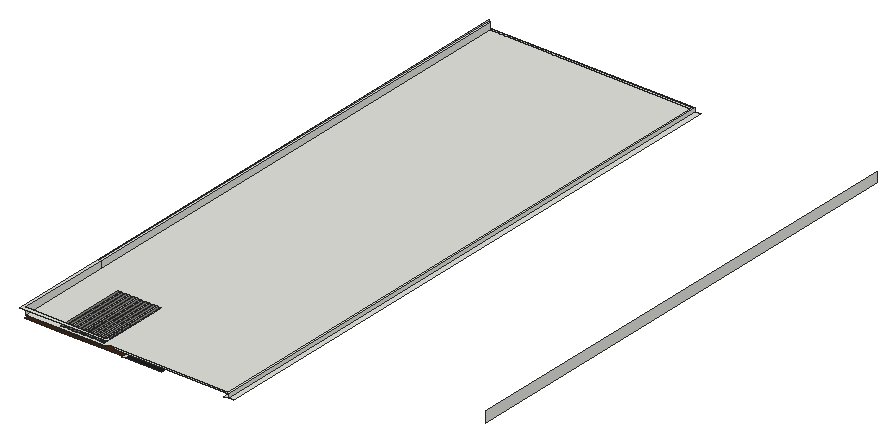
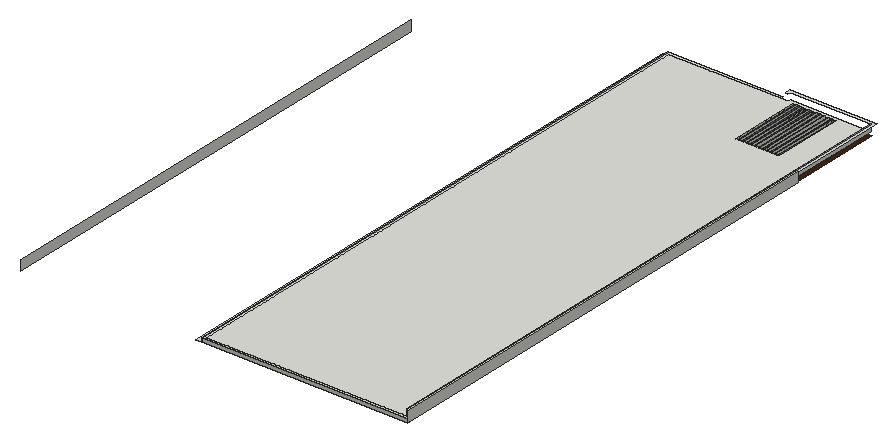
# SketchUp Ruby script. Lengths in inches.
U = 1.inch
M = Sketchup.active_model
def pt(a) = Geom::Point3d.new(a.map { |v| v * U })
def face(e, loops, mat)
  f = e.add_face(loops[0].map { |a| pt(a) })
  loops[1..].each { |l| e.add_face(l.map { |a| pt(a) }).erase! }
  f.material = f.back_material = mat if mat
  f
end
# faces: each face lists its corners as indices into pts; further lists are holes
def faces(e, pts, list, mat = nil) = list.each { |f| face(e, (f[0].is_a?(Array) ? f : [f]).map { |l| l.map { |i| pts[i] } }, mat) }
# xy, xz, yz: faces in a plane at the given z, y or x. An outline is a flat list of corners, or four numbers for a rectangle; further outlines are holes
def ring(l) = l.size == 4 ? [[l[0], l[1]], [l[2], l[1]], [l[2], l[3]], [l[0], l[3]]] : l.each_slice(2).to_a
def flat(e, list, mat, &to3) = list.each { |f| face(e, (f[0].is_a?(Array) ? f : [f]).map { |l| ring(l).map { |u, v| to3.(u, v) } }, mat) }
def xy(e, z, list, mat = nil) = flat(e, list, mat) { |x, y| [x, y, z] }
def xz(e, y, list, mat = nil) = flat(e, list, mat) { |x, z| [x, y, z] }
def yz(e, x, list, mat = nil) = flat(e, list, mat) { |y, z| [x, y, z] }
def lines(e, pts, list) = list.each { |a, b| e.add_line(pt(pts[a]), pt(pts[b])) }
# prism: a flat outline (further loops are holes) pulled along v
def prism(e, loops, v, mat = nil)
  f = face(e, loops, mat); d = Geom::Vector3d.new(v.map { |x| x * U })
  f.pushpull(f.normal.samedirection?(d) ? d.length : -d.length)
end
def box(e, o, s, mat = nil) = prism(e, [[o, [o[0] + s[0], o[1], o[2]], [o[0] + s[0], o[1] + s[1], o[2]], [o[0], o[1] + s[1], o[2]]]], [0, 0, s[2]], mat)
def at(x, y, z, deg = 0) = Geom::Transformation.translation(pt([x, y, z])) * Geom::Transformation.rotation(ORIGIN, Z_AXIS, deg.degrees)
def axes(o, x, y, z) = Geom::Transformation.new([*x, 0, *y, 0, *z, 0, *pt(o).to_a, 1])
def part(name) = M.definitions.add(name)
# library, detail: a bought-in or finely detailed component or shape, given as its bounding box
def library(name, o, s) = part(name).tap { |d| box(d.entities, o, s) }
def detail(e, o, s) = box(e.add_group.entities, o, s)
def put(e, d, t, mat = nil) = e.add_instance(d, t).tap { |i| i.material = mat if mat }
def group(e, t, mat = nil) = e.add_group.tap { |g| g.transformation = t; g.material = mat if mat }.entities
root = M.entities
M.materials.add("[Color M08]").color = [30, 30, 30]
M.materials.add("[Field Square Tile]").color = [211, 167, 108]
M.materials.add("[Granite Light Gray]").color = [149, 148, 144]
M.materials.add("[Wood Veneer 01]").color = [66, 38, 20]
xy(root,380.5,[[676.54,511.08,676.54,1825.82,228.78,1825.82,228.78,762.17,444.78,762.17,444.78,727.2,218.97,727.2,218.97,1835.625,686.35,1835.625,686.35,511.08],[444.78,511.08,453.7,589.83],[686.35,511.08,698.16,1835.625],[444.78,589.83,444.78,762.17,228.78,762.17,228.78,1825.82,676.54,1825.82,676.54,589.83,629.77,589.83,629.77,697.21,534.46,697.21,534.46,738.02,453.7,738.02,453.7,697.21,445.08,697.21,445.08,589.83],[445.08,589.83,453.7,697.21],
  [534.46,589.83,629.77,697.21],[453.7,697.21,534.46,738.02]])
xy(root,380.5,[[453.7,511.08,534.46,697.21]],"[Color M08]")
xy(root,380.5,[[[223.8,512.27,295.73,727.2],[240.83,666.01,242.35,666.38,243.73,667.14,244.86,668.22,245.67,669.56,246.1,671.0625,246.14,672.63,245.76,674.15,245.01,675.52,243.92,676.65,242.58,677.46,241.08,677.9,239.51,677.93,237.99,677.56,236.62,676.81,235.49,675.72,234.68,674.38,234.24,672.875,234.21,671.3125,234.58,669.79,235.34,668.42,236.42,667.29,237.76,666.48,239.27,666.04],[240.83,606.01,242.35,606.38,243.73,607.14,244.86,608.22,245.67,609.56,246.1,611.0625,246.14,612.63,245.76,614.15,245.01,615.52,243.92,616.65,242.58,617.46,241.08,617.9,239.51,617.93,237.99,617.56,236.62,616.81,235.49,615.72,234.68,614.38,234.24,612.875,234.21,611.3125,234.58,609.79,235.34,608.42,236.42,607.29,237.76,606.48,239.27,606.04],[240.83,554.26,242.35,554.63,243.73,555.39,244.86,556.47,245.67,557.81,246.1,559.3125,246.14,560.88,245.76,562.4,245.01,563.77,243.92,564.9,242.58,565.71,241.08,566.15,239.51,566.18,237.99,565.81,236.62,565.06,235.49,563.97,234.68,562.63,234.24,561.125,234.21,559.5625,234.58,558.04,235.34,556.67,236.42,555.54,237.76,554.73,239.27,554.29],[240.83,523.51,242.35,523.88,243.73,524.64,244.86,525.72,245.67,527.06,246.1,528.5625,246.14,530.13,245.76,531.65,245.01,533.02,243.92,534.15,242.58,534.96,241.08,535.4,239.51,535.43,237.99,535.06,236.62,534.31,235.49,533.22,234.68,531.88,234.24,530.375,234.21,528.8125,234.58,527.29,235.34,525.92,236.42,524.79,237.76,523.98,239.27,523.54],[280.58,666.01,282.1,666.38,283.48,667.14,284.61,668.22,285.42,669.56,285.85,671.0625,285.89,672.63,285.51,674.15,284.76,675.52,283.67,676.65,282.33,677.46,280.83,677.9,279.26,677.93,277.74,677.56,276.37,676.81,275.24,675.72,274.43,674.38,273.99,672.875,273.96,671.3125,274.33,669.79,275.09,668.42,276.17,667.29,277.51,666.48,279.02,666.04],[280.58,606.01,282.1,606.38,283.48,607.14,284.61,608.22,285.42,609.56,285.85,611.0625,285.89,612.63,285.51,614.15,284.76,615.52,283.67,616.65,282.33,617.46,280.83,617.9,279.26,617.93,277.74,617.56,276.37,616.81,275.24,615.72,274.43,614.38,273.99,612.875,273.96,611.3125,274.33,609.79,275.09,608.42,276.17,607.29,277.51,606.48,279.02,606.04],[280.58,554.26,282.1,554.63,283.48,555.39,284.61,556.47,285.42,557.81,285.85,559.3125,285.89,560.88,285.51,562.4,284.76,563.77,283.67,564.9,282.33,565.71,280.83,566.15,279.26,566.18,277.74,565.81,276.37,565.06,275.24,563.97,274.43,562.63,273.99,561.125,273.96,559.5625,274.33,558.04,275.09,556.67,276.17,555.54,277.51,554.73,279.02,554.29],[280.58,523.51,282.1,523.88,283.48,524.64,284.61,525.72,285.42,527.06,285.85,528.5625,285.89,530.13,285.51,531.65,284.76,533.02,283.67,534.15,282.33,534.96,280.83,535.4,279.26,535.43,277.74,535.06,276.37,534.31,275.24,533.22,274.43,531.88,273.99,530.375,273.96,528.8125,274.33,527.29,275.09,525.92,276.17,524.79,277.51,523.98,279.02,523.54]],[[295.73,512.27,444.78,727.2],[391.18,519.43,397.43,680.49],[382.06,519.43,388.31,680.49],[372.93,519.43,379.18,680.49],[363.81,519.43,370.06,680.49],[354.68,519.43,360.93,680.49],[345.56,519.43,351.81,680.49],[336.43,519.43,342.68,680.49],[327.31,519.43,333.56,680.49],[318.18,519.43,324.43,680.49],[309.06,519.43,315.31,680.49],[299.93,519.43,306.18,680.49]]],"[Wood Veneer 01]")
xy(root,381.875,[[240.83,554.26,239.27,554.29,237.76,554.73,236.42,555.54,235.34,556.67,234.58,558.04,234.21,559.5625,234.24,561.125,234.68,562.63,235.49,563.97,236.62,565.06,237.99,565.81,239.51,566.18,241.08,566.15,242.58,565.71,243.92,564.9,245.01,563.77,245.76,562.4,246.14,560.88,246.1,559.3125,245.67,557.81,244.86,556.47,243.73,555.39,242.35,554.63],[280.58,554.26,279.02,554.29,277.51,554.73,276.17,555.54,275.09,556.67,274.33,558.04,273.96,559.5625,273.99,561.125,274.43,562.63,275.24,563.97,276.37,565.06,277.74,565.81,279.26,566.18,280.83,566.15,282.33,565.71,283.67,564.9,284.76,563.77,285.51,562.4,285.89,560.88,285.85,559.3125,285.42,557.81,284.61,556.47,283.48,555.39,282.1,554.63],[240.83,606.01,239.27,606.04,237.76,606.48,236.42,607.29,235.34,608.42,234.58,609.79,234.21,611.3125,234.24,612.875,234.68,614.38,235.49,615.72,236.62,616.81,237.99,617.56,239.51,617.93,241.08,617.9,242.58,617.46,243.92,616.65,245.01,615.52,245.76,614.15,246.14,612.63,246.1,611.0625,245.67,609.56,244.86,608.22,243.73,607.14,242.35,606.38],[280.58,606.01,279.02,606.04,277.51,606.48,276.17,607.29,275.09,608.42,274.33,609.79,273.96,611.3125,273.99,612.875,274.43,614.38,275.24,615.72,276.37,616.81,277.74,617.56,279.26,617.93,280.83,617.9,282.33,617.46,283.67,616.65,284.76,615.52,285.51,614.15,285.89,612.63,285.85,611.0625,285.42,609.56,284.61,608.22,283.48,607.14,282.1,606.38],[240.83,666.01,239.27,666.04,237.76,666.48,236.42,667.29,235.34,668.42,234.58,669.79,234.21,671.3125,234.24,672.875,234.68,674.38,235.49,675.72,236.62,676.81,237.99,677.56,239.51,677.93,241.08,677.9,242.58,677.46,243.92,676.65,245.01,675.52,245.76,674.15,246.14,672.63,246.1,671.0625,245.67,669.56,244.86,668.22,243.73,667.14,242.35,666.38],
  [280.58,666.01,279.02,666.04,277.51,666.48,276.17,667.29,275.09,668.42,274.33,669.79,273.96,671.3125,273.99,672.875,274.43,674.38,275.24,675.72,276.37,676.81,277.74,677.56,279.26,677.93,280.83,677.9,282.33,677.46,283.67,676.65,284.76,675.52,285.51,674.15,285.89,672.63,285.85,671.0625,285.42,669.56,284.61,668.22,283.48,667.14,282.1,666.38]],"[Field Square Tile]")
xy(root,388.625,[[[225.31,510.87,408.63,510.87,408.63,517.43,680,517.43,680,1829.28,225.31,1829.28],[299.93,519.43,306.18,680.49],[309.06,519.43,315.31,680.49],[318.18,519.43,324.43,680.49],[327.31,519.43,333.56,680.49],[336.43,519.43,342.68,680.49],[345.56,519.43,351.81,680.49],[354.68,519.43,360.93,680.49],[363.81,519.43,370.06,680.49],[372.93,519.43,379.18,680.49],[382.06,519.43,388.31,680.49],[391.18,519.43,397.43,680.49]],[425.6875,511.08,686.35,511.08,686.35,1835.625,218.97,1835.625,225.31,1829.28,680,1829.28,680,517.43,425.6875,517.43]])
xy(root,403.8125,[[218.97,504.52,414.98,504.52,414.98,517.43,408.63,517.43,408.63,510.87,225.31,510.87,225.31,1829.28,218.97,1835.625]])
xz(root,680.49,[[299.93,380.5,306.18,388.625],[309.06,380.5,315.31,388.625],[318.18,380.5,324.43,388.625],[327.31,380.5,333.56,388.625],[336.43,380.5,342.68,388.625],
  [345.56,380.5,351.81,388.625],[354.68,380.5,360.93,388.625],[363.81,380.5,370.06,388.625],[372.93,380.5,379.18,388.625],[382.06,380.5,388.31,388.625],
  [391.18,380.5,397.43,388.625]],"[Granite Light Gray]")
xz(root,1835.625,[[218.97,380.5,686.35,388.625]])
yz(root,218.97,[[727.2,380.5,1835.625,403.8125]])
yz(root,225.31,[[510.87,388.625,727.2,403.8125],[727.2,388.625,1829.28,403.8125]])
yz(root,299.93,[[519.43,380.5,680.49,388.625]],"[Granite Light Gray]")
yz(root,306.18,[[519.43,380.5,680.49,388.625]])
yz(root,309.06,[[519.43,380.5,680.49,388.625]],"[Granite Light Gray]")
yz(root,315.31,[[519.43,380.5,680.49,388.625]])
yz(root,318.18,[[519.43,380.5,680.49,388.625]],"[Granite Light Gray]")
yz(root,324.43,[[519.43,380.5,680.49,388.625]])
yz(root,327.31,[[519.43,380.5,680.49,388.625]],"[Granite Light Gray]")
yz(root,333.56,[[519.43,380.5,680.49,388.625]])
yz(root,336.43,[[519.43,380.5,680.49,388.625]],"[Granite Light Gray]")
yz(root,342.68,[[519.43,380.5,680.49,388.625]])
yz(root,345.56,[[519.43,380.5,680.49,388.625]],"[Granite Light Gray]")
yz(root,351.81,[[519.43,380.5,680.49,388.625]])
yz(root,354.68,[[519.43,380.5,680.49,388.625]],"[Granite Light Gray]")
yz(root,360.93,[[519.43,380.5,680.49,388.625]])
yz(root,363.81,[[519.43,380.5,680.49,388.625]],"[Granite Light Gray]")
yz(root,370.06,[[519.43,380.5,680.49,388.625]])
yz(root,372.93,[[519.43,380.5,680.49,388.625]],"[Granite Light Gray]")
yz(root,379.18,[[519.43,380.5,680.49,388.625]])
yz(root,382.06,[[519.43,380.5,680.49,388.625]],"[Granite Light Gray]")
yz(root,388.31,[[519.43,380.5,680.49,388.625]])
yz(root,391.18,[[519.43,380.5,680.49,388.625]],"[Granite Light Gray]")
yz(root,397.43,[[519.43,380.5,680.49,388.625]])
yz(root,686.35,[[511.08,380.5,1835.625,388.625]])
yz(root,1097.72,[[727.2,380.5,1835.625,403.8125]])
p = [[239.27,554.29,380.5],[237.76,554.73,380.5],[237.76,554.73,381.875],[239.27,554.29,381.875],[240.83,554.26,380.5],[240.83,554.26,381.875],
  [242.35,554.63,380.5],[242.35,554.63,381.875],[279.02,554.29,380.5],[277.51,554.73,380.5],[277.51,554.73,381.875],[279.02,554.29,381.875],
  [280.58,554.26,380.5],[280.58,554.26,381.875],[282.1,554.63,380.5],[282.1,554.63,381.875],[243.73,555.39,380.5],[243.73,555.39,381.875],
  [283.48,555.39,380.5],[283.48,555.39,381.875],[236.42,555.54,380.5],[236.42,555.54,381.875],[276.17,555.54,380.5],[276.17,555.54,381.875],
  [244.86,556.47,380.5],[244.86,556.47,381.875],[284.61,556.47,380.5],[284.61,556.47,381.875],[235.34,556.67,380.5],[235.34,556.67,381.875],
  [275.09,556.67,380.5],[275.09,556.67,381.875],[245.67,557.81,380.5],[245.67,557.81,381.875],[285.42,557.81,380.5],[285.42,557.81,381.875],
  [234.58,558.04,380.5],[234.58,558.04,381.875],[274.33,558.04,380.5],[274.33,558.04,381.875],[246.1,559.3125,380.5],[246.1,559.3125,381.875],
  [285.85,559.3125,380.5],[285.85,559.3125,381.875],[234.21,559.5625,380.5],[234.21,559.5625,381.875],[273.96,559.5625,380.5],[273.96,559.5625,381.875],
  [246.14,560.88,380.5],[246.14,560.88,381.875],[285.89,560.88,380.5],[285.89,560.88,381.875],[234.24,561.125,380.5],[234.24,561.125,381.875],
  [273.99,561.125,380.5],[273.99,561.125,381.875],[245.76,562.4,380.5],[245.76,562.4,381.875],[285.51,562.4,380.5],[285.51,562.4,381.875],
  [234.68,562.63,380.5],[234.68,562.63,381.875],[274.43,562.63,380.5],[274.43,562.63,381.875],[245.01,563.77,380.5],[245.01,563.77,381.875],
  [284.76,563.77,380.5],[284.76,563.77,381.875],[235.49,563.97,380.5],[235.49,563.97,381.875],[275.24,563.97,380.5],[275.24,563.97,381.875],
  [243.92,564.9,380.5],[243.92,564.9,381.875],[283.67,564.9,380.5],[283.67,564.9,381.875],[236.62,565.06,380.5],[236.62,565.06,381.875],
  [276.37,565.06,380.5],[276.37,565.06,381.875],[242.58,565.71,380.5],[242.58,565.71,381.875],[282.33,565.71,380.5],[282.33,565.71,381.875],
  [237.99,565.81,380.5],[237.99,565.81,381.875],[277.74,565.81,380.5],[277.74,565.81,381.875],[241.08,566.15,380.5],[241.08,566.15,381.875],
  [280.83,566.15,380.5],[280.83,566.15,381.875],[239.51,566.18,380.5],[239.51,566.18,381.875],[279.26,566.18,380.5],[279.26,566.18,381.875],
  [239.27,606.04,380.5],[237.76,606.48,380.5],[237.76,606.48,381.875],[239.27,606.04,381.875],[240.83,606.01,380.5],[240.83,606.01,381.875],
  [242.35,606.38,380.5],[242.35,606.38,381.875],[279.02,606.04,380.5],[277.51,606.48,380.5],[277.51,606.48,381.875],[279.02,606.04,381.875],
  [280.58,606.01,380.5],[280.58,606.01,381.875],[282.1,606.38,380.5],[282.1,606.38,381.875],[243.73,607.14,380.5],[243.73,607.14,381.875],
  [283.48,607.14,380.5],[283.48,607.14,381.875],[236.42,607.29,380.5],[236.42,607.29,381.875],[276.17,607.29,380.5],[276.17,607.29,381.875],
  [244.86,608.22,380.5],[244.86,608.22,381.875],[284.61,608.22,380.5],[284.61,608.22,381.875],[235.34,608.42,380.5],[235.34,608.42,381.875],
  [275.09,608.42,380.5],[275.09,608.42,381.875],[245.67,609.56,380.5],[245.67,609.56,381.875],[285.42,609.56,380.5],[285.42,609.56,381.875],
  [234.58,609.79,380.5],[234.58,609.79,381.875],[274.33,609.79,380.5],[274.33,609.79,381.875],[246.1,611.0625,380.5],[246.1,611.0625,381.875],
  [285.85,611.0625,380.5],[285.85,611.0625,381.875],[234.21,611.3125,380.5],[234.21,611.3125,381.875],[273.96,611.3125,380.5],[273.96,611.3125,381.875],
  [246.14,612.63,380.5],[246.14,612.63,381.875],[285.89,612.63,380.5],[285.89,612.63,381.875],[234.24,612.875,380.5],[234.24,612.875,381.875],
  [273.99,612.875,380.5],[273.99,612.875,381.875],[245.76,614.15,380.5],[245.76,614.15,381.875],[285.51,614.15,380.5],[285.51,614.15,381.875],
  [234.68,614.38,380.5],[234.68,614.38,381.875],[274.43,614.38,380.5],[274.43,614.38,381.875],[245.01,615.52,380.5],[245.01,615.52,381.875],
  [284.76,615.52,380.5],[284.76,615.52,381.875],[235.49,615.72,380.5],[235.49,615.72,381.875],[275.24,615.72,380.5],[275.24,615.72,381.875],
  [243.92,616.65,380.5],[243.92,616.65,381.875],[283.67,616.65,380.5],[283.67,616.65,381.875],[236.62,616.81,380.5],[236.62,616.81,381.875],
  [276.37,616.81,380.5],[276.37,616.81,381.875],[242.58,617.46,380.5],[242.58,617.46,381.875],[282.33,617.46,380.5],[282.33,617.46,381.875],
  [237.99,617.56,380.5],[237.99,617.56,381.875],[277.74,617.56,380.5],[277.74,617.56,381.875],[241.08,617.9,380.5],[241.08,617.9,381.875],
  [280.83,617.9,380.5],[280.83,617.9,381.875],[239.51,617.93,380.5],[239.51,617.93,381.875],[279.26,617.93,380.5],[279.26,617.93,381.875],
  [239.27,666.04,380.5],[237.76,666.48,380.5],[237.76,666.48,381.875],[239.27,666.04,381.875],[240.83,666.01,380.5],[240.83,666.01,381.875],
  [242.35,666.38,380.5],[242.35,666.38,381.875],[279.02,666.04,380.5],[277.51,666.48,380.5],[277.51,666.48,381.875],[279.02,666.04,381.875],
  [280.58,666.01,380.5],[280.58,666.01,381.875],[282.1,666.38,380.5],[282.1,666.38,381.875],[243.73,667.14,380.5],[243.73,667.14,381.875],
  [283.48,667.14,380.5],[283.48,667.14,381.875],[236.42,667.29,380.5],[236.42,667.29,381.875],[276.17,667.29,380.5],[276.17,667.29,381.875],
  [244.86,668.22,380.5],[244.86,668.22,381.875],[284.61,668.22,380.5],[284.61,668.22,381.875],[235.34,668.42,380.5],[235.34,668.42,381.875],
  [275.09,668.42,380.5],[275.09,668.42,381.875],[245.67,669.56,380.5],[245.67,669.56,381.875],[285.42,669.56,380.5],[285.42,669.56,381.875],
  [234.58,669.79,380.5],[234.58,669.79,381.875],[274.33,669.79,380.5],[274.33,669.79,381.875],[246.1,671.0625,380.5],[246.1,671.0625,381.875],
  [285.85,671.0625,380.5],[285.85,671.0625,381.875],[234.21,671.3125,380.5],[234.21,671.3125,381.875],[273.96,671.3125,380.5],[273.96,671.3125,381.875],
  [246.14,672.63,380.5],[246.14,672.63,381.875],[285.89,672.63,380.5],[285.89,672.63,381.875],[234.24,672.875,380.5],[234.24,672.875,381.875],
  [273.99,672.875,380.5],[273.99,672.875,381.875],[245.76,674.15,380.5],[245.76,674.15,381.875],[285.51,674.15,380.5],[285.51,674.15,381.875],
  [234.68,674.38,380.5],[234.68,674.38,381.875],[274.43,674.38,380.5],[274.43,674.38,381.875],[245.01,675.52,380.5],[245.01,675.52,381.875],
  [284.76,675.52,380.5],[284.76,675.52,381.875],[235.49,675.72,380.5],[235.49,675.72,381.875],[275.24,675.72,380.5],[275.24,675.72,381.875],
  [243.92,676.65,380.5],[243.92,676.65,381.875],[283.67,676.65,380.5],[283.67,676.65,381.875],[236.62,676.81,380.5],[236.62,676.81,381.875],
  [276.37,676.81,380.5],[276.37,676.81,381.875],[242.58,677.46,380.5],[242.58,677.46,381.875],[282.33,677.46,380.5],[282.33,677.46,381.875],
  [237.99,677.56,380.5],[237.99,677.56,381.875],[277.74,677.56,380.5],[277.74,677.56,381.875],[241.08,677.9,380.5],[241.08,677.9,381.875],
  [280.83,677.9,380.5],[280.83,677.9,381.875],[239.51,677.93,380.5],[239.51,677.93,381.875],[279.26,677.93,380.5],[279.26,677.93,381.875],
  [225.31,1829.28,388.625],[218.97,1835.625,388.625],[218.97,1835.625,403.8125],[225.31,1829.28,403.8125]]
faces(root,p,[[0,1,2,3],[4,0,3,5],[6,4,5,7],[8,9,10,11],[12,8,11,13],[14,12,13,15],[16,6,7,17],[18,14,15,19],
  [1,20,21,2],[9,22,23,10],[24,16,17,25],[26,18,19,27],[20,28,29,21],[22,30,31,23],[32,24,25,33],[34,26,27,35],
  [28,36,37,29],[30,38,39,31],[40,32,33,41],[42,34,35,43],[36,44,45,37],[38,46,47,39],[48,40,41,49],[50,42,43,51],
  [44,52,53,45],[46,54,55,47],[56,48,49,57],[58,50,51,59],[52,60,61,53],[54,62,63,55],[64,56,57,65],[66,58,59,67],
  [60,68,69,61],[62,70,71,63],[72,64,65,73],[74,66,67,75],[68,76,77,69],[70,78,79,71],[80,72,73,81],[82,74,75,83],
  [76,84,85,77],[78,86,87,79],[88,80,81,89],[90,82,83,91],[84,92,93,85],[86,94,95,87],[92,88,89,93],[94,90,91,95],
  [96,97,98,99],[100,96,99,101],[102,100,101,103],[104,105,106,107],[108,104,107,109],[110,108,109,111],[112,102,103,113],[114,110,111,115],
  [97,116,117,98],[105,118,119,106],[120,112,113,121],[122,114,115,123],[116,124,125,117],[118,126,127,119],[128,120,121,129],[130,122,123,131],
  [124,132,133,125],[126,134,135,127],[136,128,129,137],[138,130,131,139],[132,140,141,133],[134,142,143,135],[144,136,137,145],[146,138,139,147],
  [140,148,149,141],[142,150,151,143],[152,144,145,153],[154,146,147,155],[148,156,157,149],[150,158,159,151],[160,152,153,161],[162,154,155,163],
  [156,164,165,157],[158,166,167,159],[168,160,161,169],[170,162,163,171],[164,172,173,165],[166,174,175,167],[176,168,169,177],[178,170,171,179],
  [172,180,181,173],[174,182,183,175],[184,176,177,185],[186,178,179,187],[180,188,189,181],[182,190,191,183],[188,184,185,189],[190,186,187,191],
  [192,193,194,195],[196,192,195,197],[198,196,197,199],[200,201,202,203],[204,200,203,205],[206,204,205,207],[208,198,199,209],[210,206,207,211],
  [193,212,213,194],[201,214,215,202],[216,208,209,217],[218,210,211,219],[212,220,221,213],[214,222,223,215],[224,216,217,225],[226,218,219,227],
  [220,228,229,221],[222,230,231,223],[232,224,225,233],[234,226,227,235],[228,236,237,229],[230,238,239,231],[240,232,233,241],[242,234,235,243],
  [236,244,245,237],[238,246,247,239],[248,240,241,249],[250,242,243,251],[244,252,253,245],[246,254,255,247],[256,248,249,257],[258,250,251,259],
  [252,260,261,253],[254,262,263,255],[264,256,257,265],[266,258,259,267],[260,268,269,261],[262,270,271,263],[272,264,265,273],[274,266,267,275],
  [268,276,277,269],[270,278,279,271],[280,272,273,281],[282,274,275,283],[276,284,285,277],[278,286,287,279],[284,280,281,285],[286,282,283,287]],"[Field Square Tile]")
faces(root,p,[[288,289,290,291]])
